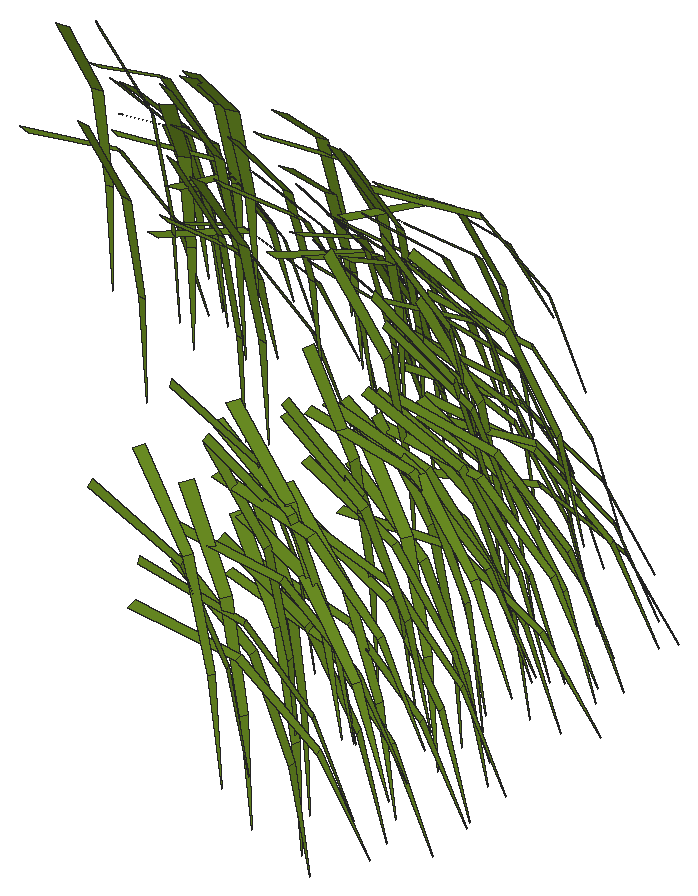
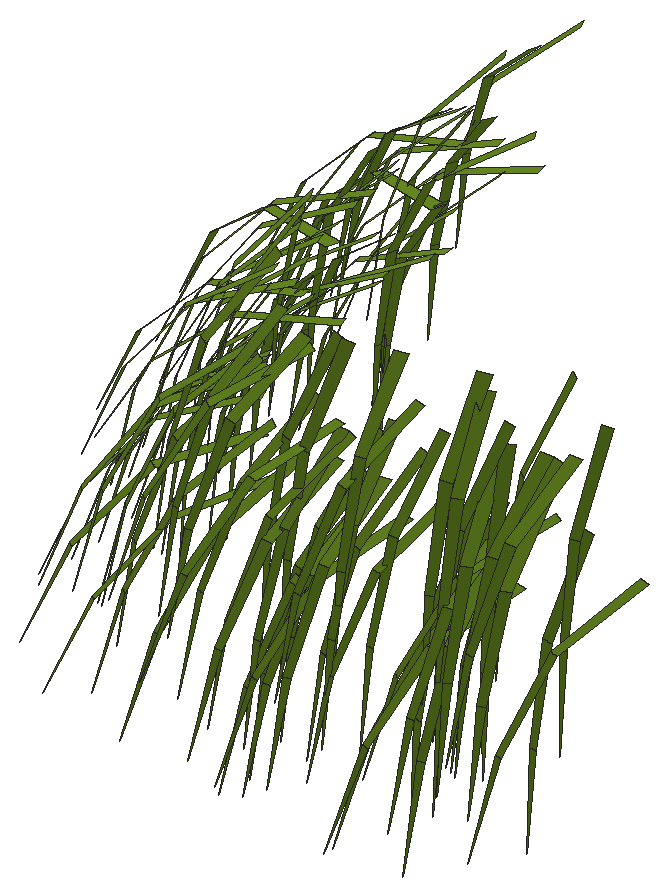
# SketchUp Ruby script. Lengths in inches.
U = 1.inch
M = Sketchup.active_model
def pt(a) = Geom::Point3d.new(a.map { |v| v * U })
def face(e, loops, mat)
  f = e.add_face(loops[0].map { |a| pt(a) })
  loops[1..].each { |l| e.add_face(l.map { |a| pt(a) }).erase! }
  f.material = f.back_material = mat if mat
  f
end
# faces: each face lists its corners as indices into pts; further lists are holes
def faces(e, pts, list, mat = nil) = list.each { |f| face(e, (f[0].is_a?(Array) ? f : [f]).map { |l| l.map { |i| pts[i] } }, mat) }
# xy, xz, yz: faces in a plane at the given z, y or x. An outline is a flat list of corners, or four numbers for a rectangle; further outlines are holes
def ring(l) = l.size == 4 ? [[l[0], l[1]], [l[2], l[1]], [l[2], l[3]], [l[0], l[3]]] : l.each_slice(2).to_a
def flat(e, list, mat, &to3) = list.each { |f| face(e, (f[0].is_a?(Array) ? f : [f]).map { |l| ring(l).map { |u, v| to3.(u, v) } }, mat) }
def xy(e, z, list, mat = nil) = flat(e, list, mat) { |x, y| [x, y, z] }
def xz(e, y, list, mat = nil) = flat(e, list, mat) { |x, z| [x, y, z] }
def yz(e, x, list, mat = nil) = flat(e, list, mat) { |y, z| [x, y, z] }
def lines(e, pts, list) = list.each { |a, b| e.add_line(pt(pts[a]), pt(pts[b])) }
# prism: a flat outline (further loops are holes) pulled along v
def prism(e, loops, v, mat = nil)
  f = face(e, loops, mat); d = Geom::Vector3d.new(v.map { |x| x * U })
  f.pushpull(f.normal.samedirection?(d) ? d.length : -d.length)
end
def box(e, o, s, mat = nil) = prism(e, [[o, [o[0] + s[0], o[1], o[2]], [o[0] + s[0], o[1] + s[1], o[2]], [o[0], o[1] + s[1], o[2]]]], [0, 0, s[2]], mat)
def at(x, y, z, deg = 0) = Geom::Transformation.translation(pt([x, y, z])) * Geom::Transformation.rotation(ORIGIN, Z_AXIS, deg.degrees)
def axes(o, x, y, z) = Geom::Transformation.new([*x, 0, *y, 0, *z, 0, *pt(o).to_a, 1])
def part(name) = M.definitions.add(name)
# library, detail: a bought-in or finely detailed component or shape, given as its bounding box
def library(name, o, s) = part(name).tap { |d| box(d.entities, o, s) }
def detail(e, o, s) = box(e.add_group.entities, o, s)
def put(e, d, t, mat = nil) = e.add_instance(d, t).tap { |i| i.material = mat if mat }
def group(e, t, mat = nil) = e.add_group.tap { |g| g.transformation = t; g.material = mat if mat }.entities
root = M.entities
M.materials.add("[0061_OliveDrab]").color = [107, 142, 35]
p = [[577.83,20.96,549.42],[577.77,20.76,549.42],[578.03,20.79,546.8],[579.23,24.125,549.35],[579.24,23.93,549.35],[579.96,24.09,546.83],
  [570.54,34.85,549.34],[570.72,34.77,549.34],[570.88,35.45,546.81],[578.74,25.56,549.44],[578.75,25.35,549.44],[579.34,25.48,546.89],
  [577.66,26.49,549.53],[577.67,26.3,549.53],[577.88,26.4,546.91],[577.51,27.23,549.49],[577.61,27.03,549.49],[577.79,27.24,546.88],
  [577.79,32.05,549.21],[577.96,31.9,549.21],[578.625,32.84,546.85],[566.39,33.86,549.55],[566.62,33.84,549.55],[566.52,34.06,546.9375],
  [570.48,34.24,549.45],[570.67,34.17,549.45],[570.72,34.5625,546.85],[566.84,35.11,549.34],[567.03,35.03,549.34],[567.3,35.87,546.86],
  [578.54,19.9,549.64],[578.57,19.68,549.64],[578.99,19.85,547.05],[575.68,33.92,549.42],[575.81,33.79,549.42],[576.56,34.625,547.05],
  [578.82,21.82,549.6875],[578.875,21.61,549.6875],[579.48,21.86,547.14],[578.03,28.03,549.66],[578.09,27.84,549.66],[578.43,28.05,547.0625],
  [575.09,33.53,549.64],[575.27,33.4,549.64],[575.625,34.05,547.125],[563.4,33.53,549.71],[563.59,33.5,549.71],[563.52,33.67,547.09],
  [566.08,33.52,549.7],[566.26,33.46,549.7],[566.22,33.64,547.08],[579.49,23.1,549.64],[579.54,22.92,549.64],[580.49,23.31,547.22],
  [577.44,21.71,549.9],[577.41,21.52,549.9],[577.6,21.59,547.28],[579.79,21.73,549.76],[579.8125,21.55,549.76],[580.82,21.75,547.34],
  [578.69,29.63,549.8],[578.77,29.43,549.8],[579.55,29.84,547.32],[564.91,35.58,549.78],[565.1,35.625,549.78],[564.77,36.53,547.34],
  [578.84,27.42,549.85],[578.91,27.22,549.85],[579.64,27.59,547.35],[578.67,29,549.9],[578.6875,28.82,549.9],[579.47,28.99,547.4],
  [578.42,24.73,550.08],[578.35,24.54,550.08],[578.77,24.48,547.48],[578.9,22.46,550.11],[578.86,22.28,550.11],[579.45,22.22,547.55],
  [579.64,24.29,549.98],[579.68,24.11,549.98],[580.68,24.4,547.57],[577.02,31.1,550.14],[577.14,30.95,550.14],[577.55,31.41,547.58],
  [566.11,36.09,549.9375],[566.3125,36.04,549.9375],[566.49,37.19,547.59],[578.3125,31.02,550.08],[578.39,30.83,550.08],[579.3,31.33,547.67],
  [576.81,31.34,550.26],[576.95,31.18,550.26],[577.29,31.6,547.6875],[572.76,35.22,550.1],[572.98,35.15,550.1],[573.16,36.12,547.66],
  [578.01,31.4,550.29],[578.17,31.23,550.29],[578.78,31.98,547.85],[575.39,32.76,550.46],[575.57,32.65,550.46],[575.7,33.07,547.87],
  [570.38,34.625,550.51],[570.57,34.61,550.51],[570.5,35.04,547.92],[569.16,35.8,550.35],[569.35,35.81,550.35],[569.23,36.67,547.875],
  [569.85,34.07,550.5625],[570.03,34.01,550.5625],[570.03,34.3,547.95],[568,35,550.59],[568.2,34.92,550.59],[568.32,35.53,548.03],
  [562.87,35.42,550.53],[563.05,35.36,550.53],[563.23,36.14,548.02],[568.6875,34.4,550.65],[568.88,34.33,550.65],[568.92,34.76,548.05],
  [568.71,35.61,550.59],[568.91,35.62,550.59],[568.77,36.38,548.08],[569.33,36.03,550.51],[569.53,35.98,550.51],[569.7,37.08,548.13],
  [579.29,24.45,550.66],[579.31,24.27,550.66],[580.17,24.49,548.19],[576.54,29.55,550.8125],[576.59,29.35,550.8125],[576.75,29.49,548.2],
  [571.16,34.74,550.73],[571.33,34.67,550.73],[571.44,35.15,548.15],[570.62,35.67,550.67],[570.83,35.66,550.67],[570.79,36.66,548.24],
  [580.15,26.35,550.58],[580.2,26.16,550.58],[581.48,26.62,548.33],[578.93,20.07,550.86],[579.03,19.9,550.86],[579.74,20.41,548.39],
  [578.05,18.94,551.05],[577.97,18.75,551.05],[578.33,18.71,548.45],[580,18.97,550.86],[580.05,18.76,550.86],[581.21,19.12,548.53],
  [578.84,27.6,550.99],[578.91,27.4,550.99],[579.61,27.76,548.48],[578.8,25.53,551.18],[578.82,25.34,551.18],[579.29,25.48,548.6],
  [567.4375,34.26,551.21],[567.62,34.25,551.21],[567.55,34.59,548.61],[564.93,35.93,551],[565.13,35.96,551],[564.875,36.95,548.57],
  [564.63,33.63,551.28],[564.8125,33.71,551.28],[564.62,33.89,548.66],[571.96,34.66,551.22],[572.16,34.6,551.22],[572.23,35.21,548.66],
  [577.61,21,551.37],[577.63,20.82,551.37],[577.83,20.93,548.75],[576.48,32.57,551.29],[576.625,32.42,551.29],[577.03,32.95,548.75],
  [568.11,34.78,551.41],[568.29,34.82,551.41],[568.11,35.26,548.83],[579.06,26.95,551.4],[579.125,26.74,551.4],[579.76,27.05,548.87],
  [566.02,35.15,551.36],[566.18,35.05,551.36],[566.51,35.78,548.85],[578.69,23.66,551.55],[578.71,23.45,551.55],[579.27,23.61,548.99],
  [578.21,23.97,551.5625],[578.26,23.78,551.5625],[578.62,23.97,548.97],[566.01,33.55,551.65],[566.23,33.5,551.65],[566.17,33.71,549.04],
  [564.79,34.26,551.64],[564.98,34.21,551.64],[564.98,34.58,549.04],[563.44,35.24,551.54],[563.64,35.3,551.54],[563.36,35.98,549.02],
  [579.41,28.23,551.5],[579.47,28.03,551.5],[580.4,28.44,549.08],[564.6,35.01,551.64],[564.79,35.08,551.64],[564.45,35.72,549.12],
  [577.87,28.28,551.81],[577.95,28.11,551.81],[578.3,28.38,549.22],[576.54,30.67,551.07],[576.78,30.47,551.07],[564.5,34.47,551.77],
  [564.72,34.46,551.77],[564.62,34.86,549.17],[577.9,24.04,551.61],[577.92,23.77,551.61],[580.04,26.92,551.65],[580.05,26.72,551.65],
  [581.18,26.91,549.29],[571.29,33.1,551.95],[571.5,33.03,551.95],[571.45,33.23,549.33],[570.0625,33.73,551.67],[570.32,33.63,551.67],
  [566.21,33.84,551.54],[566.47,33.72,551.54],[577.25,21.18,551.97],[577.17,20.9,551.97],[578.37,21.56,552.02],[578.42,21.38,552.02],
  [578.84,21.6,549.44],[577.35,24.12,551.98],[577.33,23.93,551.98],[577.52,24,549.37],[577.63,25.5625,551.82],[577.64,25.27,551.82],
  [574.375,32.75,551.375],[574.56,32.56,551.375],[570.45,33.42,552.01],[570.67,33.41,552.01],[570.57,33.62,549.4],[577.09,26.51,552.09],
  [577.11,26.23,552.09],[576.93,26.99,552.04],[577.07,26.71,552.04],[575.8,31.03,552.05],[575.98,30.91,552.05],[576.08,31.27,549.45],
  [570.12,33.49,551.9375],[570.39,33.375,551.9375],[577.59,19.82,552.08],[577.63,19.51,552.08],[579.83,20.54,551.98],[579.88,20.35,551.98],
  [580.92,20.73,549.6],[577.92,22.65,551.7],[577.99,22.4,551.7],[574.26,32.52,551.92],[574.51,32.33,551.92],[566.3,33.29,552.11],
  [566.62,33.26,552.11],[577.65,21.59,552.03],[577.73,21.28,552.03],[579.48,25.57,552.16],[579.53,25.35,552.16],[580.38,25.68,549.7],
  [577.19,27.82,552.14],[577.28,27.54,552.14],[577.28,28.14,552.34],[577.39,27.94,552.34],[577.59,28.19,549.74],[563.29,33.09,552.29],
  [563.5625,33.05,552.29],[565.9,33.1,552.29],[566.16,33.02,552.29],[562.76,33.21,552.32],[562.94,33.23,552.32],[562.83,33.38,549.7],
  [573.59,33.52,552.29],[573.78,33.48,552.29],[573.77,33.98,549.71],[580.125,20.16,552.05],[580.05,19.95,552.05],[581.34,19.61,549.79],
  [578.12,21.6,551.78],[578.15,21.34,551.78],[577.57,27.01,552.11],[577.67,26.72,552.11],[577.31,29.16,551.98],[577.42,28.87,551.98],
  [565.25,34.05,551.89],[565.52,34.12,551.89],[576.98,21.83,552.48],[576.93,21.56,552.48],[577.27,28.9,552.12],[577.3,28.64,552.12],
  [565.63,34.31,551.8125],[565.91,34.24,551.8125],[568.85,35.11,552.44],[569.05,35.06,552.44],[569.09,35.71,549.89],[578.09,18.23,552.58],
  [578.18,18.05,552.58],[578.55,18.34,549.99],[578.89,20.875,552.6],[578.875,20.69,552.6],[579.48,20.73,550.05],[578.01,24.02,552.02],
  [578.06,23.77,552.02],[575.95,29.34,552.61],[576.07,29.16,552.61],[576.18,29.37,549.99],[577.375,30.41,552.61],[577.44,30.2,552.61],
  [577.95,30.47,550.05],[578.22,17.6,552.71],[578.16,17.43,552.71],[578.59,17.37,550.12],[577.78,22.78,552.46],[577.72,22.53,552.46],
  [577.58,25.11,552.53],[577.47,24.85,552.53],[576.73,30.4,552.09],[576.85,30.13,552.09],[576.11,30.43,552.51],[576.28,30.22,552.51],
  [572.24,33.72,552.2],[572.55,33.63,552.2],[572.32,34.625,552.66],[572.54,34.58,552.66],[572.54,35.2,550.11],[578.75,20.77,552.77],
  [578.6875,20.58,552.77],[579.37,20.48,550.24],[565.33,34.27,552.8125],[565.54,34.34,552.8125],[565.29,34.74,550.23],[579.84,24.93,552.66],
  [579.89,24.72,552.66],[580.98,25.06,550.29],[576.79,30.29,552.33],[577.01,30.06,552.33],[575.96,30.69,552.66],[576.16,30.46,552.66],
  [565.27,32.3,552.875],[565.42,32.1875,552.875],[565.44,32.37,550.26],[565.97,33.9375,552.91],[566.19,33.98,552.91],[566.01,34.3125,550.31],
  [568.17,34.35,552.93],[568.37,34.39,552.93],[568.18,34.79,550.34],[563.71,35.37,552.79],[563.93,35.36,552.79],[563.83,36.17,550.29],
  [571.21,36.19,552.61],[571.39,36.16,552.61],[571.55,37.4375,550.32],[569.16,34.25,552.47],[569.4375,34.26,552.47],[580.12,20.96,552.81],
  [580.12,20.76,552.81],[581.3,20.87,550.46],[576.4,26.57,553.16],[576.45,26.35,553.16],[576.61,26.5,550.54],[574.85,31.95,552.9],
  [575.1,31.8,552.9],[570.29,33.69,552.96],[570.56,33.67,552.96],[562.34,34.08,552.72],[562.59,33.99,552.72],[568.86,34.3,552.43],
  [569.14,34.23,552.43],[573.71,34.54,552.95],[573.89,34.41,552.95],[574.27,35.14,550.45],[577.2,21.72,553.21],[577.3,21.56,553.21],
  [577.55,21.84,550.61],[578.17,25.84,552.23],[578.25,25.5625,552.23],[569.58,33.44,553.1],[569.84,33.35,553.1],[568.36,33.57,553.12],
  [568.63,33.48,553.12],[567.53,33.89,552.92],[567.82,33.78,552.92],[568.76,34.18,552.79],[569.04,34.19,552.79],[580.23,24.05,552.88],
  [580.17,23.84,552.88],[581.54,23.53,550.66],[577.85,24.28,552.86],[577.89,24.02,552.86],[570.71,33.79,553.14],[570.95,33.68,553.14],
  [570.77,33.92,552.8],[570.48,34.0625,552.74],[570.78,34.04,552.74],[576.02,29.47,553.38],[576.09,29.18,553.38],[578.15,18.61,552.6875],
  [578.21,18.3125,552.6875],[577.625,19.38,553.03],[577.76,19.14,553.03],[577.57,27.2,553.25],[577.67,26.92,553.25],[565.16,34.25,553],
  [565.4375,34.29,553],[577.32,19.29,553.55],[577.21,19.02,553.55],[574.84,28.76,551.64],[575.13,28.51,551.64],[577.77,25.48,553.59],
  [577.79,25.21,553.59],[567.36,33.49,553.71],[567.61,33.47,553.71],[571.6,33.5625,553.57],[571.88,33.48,553.57],[575.53,31.74,553.59],
  [575.73,31.52,553.59],[564.85,33.04,553.83],[565.11,33.16,553.83],[577.04,20.98,553.93],[577.0625,20.72,553.93],[577.79,26.625,553.68],
  [577.88,26.32,553.68],[572.58,31.11,552.36],[572.81,30.86,552.36],[565.23,33.92,553.54],[565.45,33.79,553.54],[568.26,33.78,553.84],
  [568.52,33.83,553.84],[577.59,23.6,553.93],[577.62,23.29,553.93],[577.8,27.77,553.53],[577.89,27.49,553.53],[565.29,31.9,553.06],
  [565.61,31.76,553.06],[563.73,33.94,553.8],[564.02,34.02,553.8],[575.69,23.88,553.02],[575.72,23.54,553.02],[577.34,23.82,554.03],
  [577.41,23.55,554.03],[564.55,33.47,554.13],[564.81,33.4,554.13],[565,33.77,553.92],[565.27,33.87,553.92],[575.66,21.99,552.86],
  [575.75,21.68,552.86],[578.17,26.81,553.49],[578.19,26.52,553.49],[569.3125,31.89,553.38],[569.63,31.77,553.38],[565.84,33.04,554.22],
  [566.15,32.97,554.22],[575.69,21.375,552.74],[575.72,21.06,552.74],[575.7,25.53,553.6],[575.71,25.17,553.6],[576.99,27.92,554.26],
  [577.11,27.67,554.26],[564.99,31.87,552.55],[565.34,31.79,552.55],[564.4375,33.58,554.24],[564.74,33.57,554.24],[572.94,30.83,553.4375],
  [573.25,30.6,553.4375],[565.79,31.79,553.11],[566.125,31.87,553.11],[569.43,31.9,553.91],[569.75,31.76,553.91],[571.09,32.65,554.53],
  [571.39,32.55,554.53],[578.1,20.13,553.91],[578.17,19.86,553.91],[575.66,21.14,553.68],[575.75,20.77,553.68],[575.76,21.67,554.07],
  [575.65,21.32,554.07],[577.4,21.32,554.45],[577.47,21.07,554.45],[575.68,23.61,553.14],[575.74,23.3,553.14],[576.84,24.22,554.56],
  [576.81,23.95,554.56],[575.58,26.36,554.2],[575.75,26.01,554.2],[575.19,28.4,553.33],[575.33,28.04,553.33],[570.375,32.86,554.58],
  [570.69,32.85,554.58],[575.68,19.6,553.87],[575.73,19.22,553.87],[578.22,20.88,553.71],[578.11,20.58,553.71],[575.61,26.33,553.72],
  [575.73,25.98,553.72],[575.64,26.47,554.27],[575.65,26.14,554.27],[575.42,27.31,554.01],[575.53,26.97,554.01],[575.03,28.71,553.47],
  [575.06,28.39,553.47],[574.47,29.47,553.03],[574.6,29.14,553.03],[575.32,30.37,554.55],[575.59,30.2,554.55],[566.15,31.84,554.3],
  [566.54,31.8125,554.3],[575.66,25.16,552.58],[575.75,24.83,552.58],[577.96,25.25,554.28],[578.03,24.94,554.28],[571.51,31.52,553.42],
  [571.88,31.4,553.42],[576.61,27.79,554.86],[576.77,27.52,554.86],[574.97,28.59,553.18],[575.24,28.3125,553.18],[563.08,31.85,554.6],
  [563.41,31.8,554.6],[565.48,31.88,554.57],[565.8,31.78,554.57],[573.35,32.48,554.6875],[573.62,32.43,554.6875],[562.77,32.72,554.9],
  [563.04,32.75,554.9],[568.21,31.87,553.19],[568.56,31.78,553.19],[568.52,33.89,554.74],[568.8,33.82,554.74],[575.73,22.07,554.78],
  [575.68,21.73,554.78],[575.75,23.33,554.02],[575.67,23.02,554.02],[575.77,25.87,554.28],[575.64,25.55,554.28],[574.57,29.23,554.26],
  [574.78,28.97,554.26],[569.19,31.82,553.47],[569.53,31.83,553.47],[577.18,17.85,555.01],[577.31,17.58,555.01],[577.69,21.02,554.93],
  [577.67,20.76,554.93],[575.46,29.05,555.17],[575.64,28.8,555.17],[576.24,30.09,554.96],[576.34,29.79,554.96],[570.78,34.27,554.34],
  [571.04,34.22,554.34],[577.33,17.96,555.15],[577.24,17.72,555.15],[575.67,18.11,553.375],[575.75,17.74,553.375],[578.08,24.61,554.57],
  [578.14,24.3,554.57],[574.42,29.45,554.375],[574.65,29.17,554.375],[570.3,31.72,553.9],[570.67,31.69,553.9],[561.5,31.88,553.89],
  [561.81,31.77,553.89],[572.05,33.43,554.98],[572.35,33.37,554.98],[577.55,21.18,555.07],[577.46,20.9,555.07],[578.25,20.98,554.65],
  [578.25,20.69,554.65],[568.87,31.82,553.94],[569.21,31.84,553.94],[565.6,33.33,555.24],[565.9,33.43,555.24],[563.63,33.94,554.99],
  [563.94,33.93,554.99],[575.68,23.99,554.3],[575.73,23.67,554.3],[578.25,24.72,554.47],[578.15,24.41,554.47],[573.78,30.25,554.58],
  [574.08,30.07,554.58],[564.97,31.97,555.46],[565.18,31.81,555.46],[566.74,31.9,554.43],[567.1,31.76,554.43],[566.09,33.1,555.4],
  [566.41,33.17,555.4],[572.8125,33.35,555.11],[573.07,33.17,555.11],[568.33,33.39,555.37],[568.61,33.45,555.37],[575.625,18.3,554.35],
  [575.79,18.01,554.35],[570.15,31.75,554.72],[570.48,31.73,554.72],[565.51,31.8,553.88],[565.86,31.86,553.88],[569.84,31.87,554.7],
  [570.13,31.74,554.7],[567.75,31.88,555.03],[568.08,31.77,555.03],[569,31.88,555.125],[569.31,31.77,555.125],[576.47,21.28,555.7],
  [576.62,21.06,555.7],[575.875,26.5,555.73],[575.9375,26.2,555.73],[575.57,26.52,554.81],[575.69,26.18,554.81],[574.625,29.15,555.59],
  [574.72,28.8,555.59],[575.6,26.625,553.99],[575.63,26.27,553.99],[575.47,27.06,554.5],[575.58,26.72,554.5],[563.98,31.91,554.67],
  [564.25,31.75,554.67],[575.73,19.98,555.52],[575.6,19.66,555.52],[575.69,25.32,555.19],[575.72,24.99,555.19],[573.88,30.24,554.98],
  [574.12,29.98,554.98],[571,31.62,555.23],[571.35,31.52,555.23],[575.77,21.78,554.02],[575.64,21.42,554.02],[575.65,26.03,555.08],
  [575.76,25.66,555.08],[567.23,31.77,555.69],[567.54,31.75,555.69],[565.47,31.63,555.95],[565.79,31.78,555.95],[564.25,31.78,555.2],
  [564.61,31.875,555.2],[568.625,31.77,555.48],[568.94,31.83,555.48],[575.66,19.53,554.6875],[575.75,19.19,554.6875],[575.54,20.85,556.08],
  [575.57,20.53,556.08],[575.62,23.43,555.66],[575.66,23.05,555.66],[565.6875,31.75,555.44],[566.02,31.87,555.44],[575.55,23.45,555.92],
  [575.625,23.12,555.92],[564.0625,31.73,556.04],[564.38,31.65,556.04],[565.48,31.66,556.42],[565.85,31.57,556.42],[564.36,31.6875,556.06],
  [564.73,31.68,556.06],[575.64,24.73,555.41],[575.74,24.35,555.41],[575.26,27.15,556.07],[575.4,26.84,556.07],[570.24,31.75,554.86],
  [570.56,31.69,554.86],[575.49,20.8125,556.18],[575.58,20.5,556.18],[575.76,25.53,554.72],[575.65,25.16,554.72],[574.34,28.88,556.48],
  [574.66,28.68,556.48],[570.61,31.36,556.76],[570.98,31.24,556.76],[575.7,20.98,555.29],[575.71,20.63,555.29],[575.64,24.13,555.44],
  [575.72,23.76,555.44],[575.44,24.42,556.77],[575.4,24.1,556.77],[570.26,31.38,556.74],[570.66,31.36,556.74],[572.9375,30.43,556.27],
  [573.27,30.37,556.27],[567.99,31.71,556.11],[568.33,31.63,556.11],[575.51,21.24,556.375],[575.48,20.92,556.375],[575.1,26.93,556.82],
  [575.29,26.6,556.82],[562.9,31.35,557.14],[563.22,31.39,557.14],[575.36,17.01,556.7],[575.51,16.68,556.7],[574.14,29.46,556.4],
  [574.26,29.09,556.4],[571.59,31.24,556.35],[571.97,31.17,556.35],[563.54,31.65,556.26],[563.92,31.64,556.26],[575.51,21.83,556.59],
  [575.4,21.49,556.59],[571.4,31.4,556.16],[571.71,31.18,556.16],[575.46,18.68,556.85],[575.35,18.38,556.85],[574.24,28.24,557.35],
  [574.45,27.9375,557.35],[566.21,31.43,556.96],[566.5625,31.55,556.96],[566.43,31.26,557.24],[566.81,31.34,557.24],[568.72,31.4,557.04],
  [569.07,31.47,557.04],[564.23,31.03,557.8],[564.49,30.83,557.8],[574.89,20.28,557.53],[575.07,20,557.53],[574.47,26.24,557.93],
  [574.55,25.87,557.93]]
faces(root,p,[[0,1,2],[3,4,5],[6,7,8],[9,10,11],[12,13,14],[15,16,17],[18,19,20],[21,22,23],
  [24,25,26],[27,28,29],[30,31,32],[33,34,35],[36,37,38],[39,40,41],[42,43,44],[45,46,47],
  [48,49,50],[51,52,53],[54,55,56],[57,58,59],[60,61,62],[63,64,65],[66,67,68],[69,70,71],
  [72,73,74],[75,76,77],[78,79,80],[81,82,83],[84,85,86],[87,88,89],[90,91,92],[93,94,95],
  [96,97,98],[99,100,101],[102,103,104],[105,106,107],[108,109,110],[111,112,113],[114,115,116],[117,118,119],
  [120,121,122],[123,124,125],[126,127,128],[129,130,131],[132,133,134],[135,136,137],[138,139,140],[141,142,143],
  [144,145,146],[147,148,149],[150,151,152],[153,154,155],[156,157,158],[159,160,161],[162,163,164],[165,166,167],
  [168,169,170],[171,172,173],[174,175,176],[177,178,179],[180,181,182],[183,184,185],[186,187,188],[189,190,191],
  [192,193,194],[195,196,197],[198,199,200],[201,202,203],[204,205,206],[207,208,19,18],[209,210,211],[212,213,4,3],
  [214,215,216],[217,218,219],[220,221,7,6],[222,223,28,27],[224,225,1,0],[226,227,228],[229,230,231],[232,233,10,9],
  [234,235,34,33],[236,237,238],[239,240,13,12],[241,242,16,15],[243,244,245],[246,247,25,24],[248,249,31,30],[250,251,252],
  [253,254,52,51],[255,256,43,42],[257,258,22,21],[259,260,37,36],[261,262,263],[264,265,40,39],[266,267,268],[269,270,46,45],
  [271,272,49,48],[273,274,275],[276,277,278],[279,280,281],[282,283,58,57],[284,285,67,66],[286,287,61,60],[288,289,64,63],
  [290,291,55,54],[292,293,70,69],[294,295,85,84],[296,297,298],[299,300,301],[302,303,304],[305,306,79,78],[307,308,309],
  [310,311,312],[313,314,315],[316,317,76,75],[318,319,73,72],[320,321,88,87],[322,323,82,81],[324,325,94,93],[326,327,328],
  [329,330,331],[332,333,334],[335,336,337],[338,339,97,96],[340,341,91,90],[342,343,344],[345,346,347],[348,349,350],
  [351,352,353],[354,355,356],[357,358,106,105],[359,360,361],[362,363,364],[365,366,100,99],[367,368,103,102],[369,370,115,114],
  [371,372,124,123],[373,374,375],[376,377,378],[379,380,139,138],[381,382,109,108],[383,384,118,117],[385,386,112,111],[387,388,121,120],
  [389,390,391],[392,393,127,126],[394,395,133,132,396],[397,398,136,135],[399,400,130,129],[401,402,148,147],[403,404,142,141],[405,406,151,150],
  [407,408,160,159],[409,410,145,144],[411,412,208,207],[413,414,154,153],[415,416,157,156],[417,418,166,165],[419,420,172,171],[421,422,163,162],
  [423,424,169,168],[425,426,178,177],[427,428,235,234],[429,430,181,180],[431,432,175,174],[433,434,184,183],[435,436,199,198],[437,438,223,222],
  [439,440,196,195],[441,442,213,212],[443,444,187,186],[445,446,193,192],[447,448,202,201],[449,450,254,253],[451,452,215,214],[453,454,221,220],
  [455,456,190,189],[457,458,283,282],[459,460,233,232],[461,462,205,204],[463,464,295,294],[465,466,210,209],[467,468,256,255],[469,470,289,288],
  [471,472,247,246],[473,474,218,217],[475,476,251,250],[477,478,260,259],[479,480,225,224],[481,482,227,226],[483,484,306,305],[485,486,230,229],
  [487,488,242,241],[489,490,287,286],[491,492,237,236],[493,494,249,248],[495,496,280,279],[497,498,285,284],[499,500,240,239],[501,502,265,264],
  [503,504,293,292],[505,506,321,320],[507,508,244,243],[509,510,258,257],[511,512,380,379],[513,514,262,261],[515,516,325,324],[517,518,267,266],
  [519,520,339,338],[521,522,270,269],[523,524,272,271],[525,526,277,276],[527,528,274,273],[529,530,372,371],[531,532,297,296],[533,534,291,290],
  [535,536,317,316],[537,538,319,318],[539,540,323,322],[541,542,358,357],[543,544,300,299],[545,546,303,302],[547,548,308,307],[549,550,311,310],
  [551,552,355,354],[553,554,314,313],[555,556,402,401],[557,558,336,335],[559,560,341,340],[561,562,396,398,397],[563,564,370,369],[565,566,327,326],
  [567,568,330,329],[569,570,360,359],[571,572,388,387],[573,574,333,332],[575,576,352,351],[577,578,393,392],[579,580,390,389],[581,582,366,365],
  [583,584,343,342],[585,586,386,385],[587,588,346,345],[589,590,374,373],[591,592,349,348],[593,594,404,403],[595,596,368,367],[597,598,408,407],
  [599,600,395,394],[601,602,384,383],[603,604,382,381],[605,606,377,376],[607,608,363,362],[609,610,406,405],[611,612,400,399],[613,614,452,451],
  [615,616,436,435],[617,618,430,429],[619,620,410,409],[621,622,414,413],[623,624,420,419],[625,626,418,417],[627,628,496,495],[629,630,426,425],
  [631,632,416,415],[633,634,422,421],[635,636,440,439],[637,638,432,431],[639,640,476,475],[641,642,424,423],[643,644,434,433],[645,646,448,447],
  [647,648,444,443],[649,650,446,445],[651,652,456,455],[653,654,466,465],[655,656,514,513],[657,658,462,461],[659,660,552,551],[661,662,482,481],
  [663,664,580,579],[665,666,508,507],[667,668,474,473],[669,670,570,569],[671,672,558,557],[673,674,486,485],[675,676,492,491],[677,678,526,525],
  [679,680,532,531],[681,682,546,545],[683,684,518,517],[685,686,528,527],[687,688,544,543],[689,690,550,549],[691,692,566,565],[693,694,576,575],
  [695,696,568,567],[697,698,590,589],[699,700,554,553],[701,702,548,547],[703,704,574,573],[705,706,588,587],[707,708,592,591],[709,710,584,583],
  [711,712,606,605],[713,714,608,607]],"[0061_OliveDrab]")
